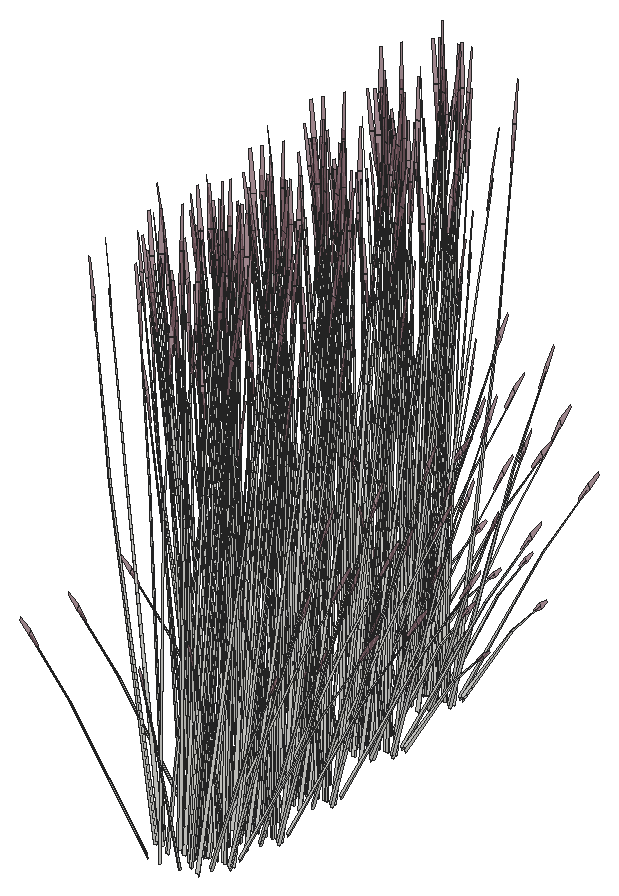
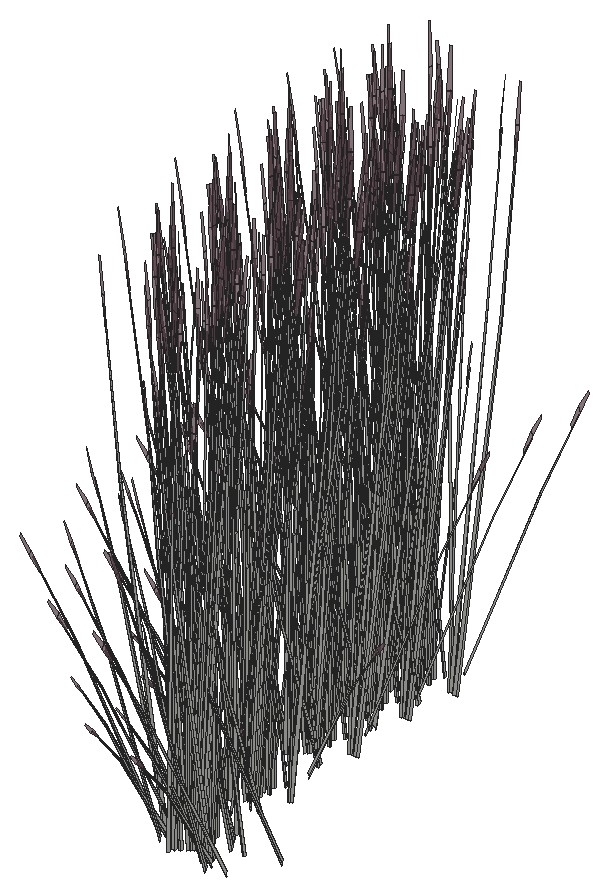
# SketchUp Ruby script. Lengths in inches.
U = 1.inch
M = Sketchup.active_model
def pt(a) = Geom::Point3d.new(a.map { |v| v * U })
def face(e, loops, mat)
  f = e.add_face(loops[0].map { |a| pt(a) })
  loops[1..].each { |l| e.add_face(l.map { |a| pt(a) }).erase! }
  f.material = f.back_material = mat if mat
  f
end
# faces: each face lists its corners as indices into pts; further lists are holes
def faces(e, pts, list, mat = nil) = list.each { |f| face(e, (f[0].is_a?(Array) ? f : [f]).map { |l| l.map { |i| pts[i] } }, mat) }
# xy, xz, yz: faces in a plane at the given z, y or x. An outline is a flat list of corners, or four numbers for a rectangle; further outlines are holes
def ring(l) = l.size == 4 ? [[l[0], l[1]], [l[2], l[1]], [l[2], l[3]], [l[0], l[3]]] : l.each_slice(2).to_a
def flat(e, list, mat, &to3) = list.each { |f| face(e, (f[0].is_a?(Array) ? f : [f]).map { |l| ring(l).map { |u, v| to3.(u, v) } }, mat) }
def xy(e, z, list, mat = nil) = flat(e, list, mat) { |x, y| [x, y, z] }
def xz(e, y, list, mat = nil) = flat(e, list, mat) { |x, z| [x, y, z] }
def yz(e, x, list, mat = nil) = flat(e, list, mat) { |y, z| [x, y, z] }
def lines(e, pts, list) = list.each { |a, b| e.add_line(pt(pts[a]), pt(pts[b])) }
# prism: a flat outline (further loops are holes) pulled along v
def prism(e, loops, v, mat = nil)
  f = face(e, loops, mat); d = Geom::Vector3d.new(v.map { |x| x * U })
  f.pushpull(f.normal.samedirection?(d) ? d.length : -d.length)
end
def box(e, o, s, mat = nil) = prism(e, [[o, [o[0] + s[0], o[1], o[2]], [o[0] + s[0], o[1] + s[1], o[2]], [o[0], o[1] + s[1], o[2]]]], [0, 0, s[2]], mat)
def at(x, y, z, deg = 0) = Geom::Transformation.translation(pt([x, y, z])) * Geom::Transformation.rotation(ORIGIN, Z_AXIS, deg.degrees)
def axes(o, x, y, z) = Geom::Transformation.new([*x, 0, *y, 0, *z, 0, *pt(o).to_a, 1])
def part(name) = M.definitions.add(name)
# library, detail: a bought-in or finely detailed component or shape, given as its bounding box
def library(name, o, s) = part(name).tap { |d| box(d.entities, o, s) }
def detail(e, o, s) = box(e.add_group.entities, o, s)
def put(e, d, t, mat = nil) = e.add_instance(d, t).tap { |i| i.material = mat if mat }
def group(e, t, mat = nil) = e.add_group.tap { |g| g.transformation = t; g.material = mat if mat }.entities
root = M.entities
M.materials.add("LightPink_Translucent").color = [144, 107, 117]
M.materials["LightPink_Translucent"].alpha = 0.75
c1 = part("blade")
p = [[2.15,0.21,22],[0,0.17,0],[0.09,0.45,0],[2.18,0.31,22],[2.29,0.31,22],[0.38,0.45,0],
  [2.48,0.24,33],[2.49,0.24,33],[2.48,0.22,33]]
faces(c1.entities,p,[[0,1,2,3],[4,5,2,3],[6,3,4,7],[8,0,3,6]])
c2 = part("seeds")
p = [[0.3,-0.1,1.38],[-0.01,-0.03,1.59],[-0.01,-0.03,0.03],[0.14,-0.07,-0.07],[0.29,-0.03,3],[0.15,0.01,3.11]]
faces(c2.entities,p,[[0,1,2,3],[1,0,4,5]],"LightPink_Translucent")
c3 = part("blade with seeds")
put(c3.entities,c1,at(0,0,0))
put(c3.entities,c2,axes([2.4,0.25,30.99],[1.5799,-0.05474,1.17369],[-0.12525,1.92788,0.29478],[-0.07173,-0.02425,1.56792]))
put(root,c3,axes([684.41,330.09,265.93],[-0.60515,0.48003,0.25528],[-0.60552,-0.47498,-0.30288],[-0.02113,-0.13632,1.36855]))
put(root,c3,axes([686.64,317.69,265.97],[-0.40676,0.57214,0],[-0.68052,-0.31907,-0.42834],[-0.15499,-0.07267,1.3588]))
put(root,c3,axes([685.4375,325.0625,266.15],[0.2053,-0.09007,1.18691],[0.50689,0.27159,-0.25526],[-0.15087,0.235,0.50747]))
put(root,c3,axes([685.47,313.58,266.15],[0.2053,-0.09007,1.18691],[0.50689,0.27159,-0.25526],[-0.15087,0.235,0.50747]))
put(root,c3,axes([684.76,327.24,266.3],[0.33937,0.19872,0.95334],[-0.49424,0.11946,0.70045],[-0.10575,-0.15273,0.20998]))
put(root,c3,axes([683.1875,341.02,266.34],[0.59102,-0.10111,0.05401],[0.13587,0.40735,-0.71633],[-0.03747,0.2062,0.64209]))
put(root,c3,axes([686.01,319.34,266.15],[-0.0394,0.18678,1.18691],[-0.57594,0.15636,-0.25526],[-0.13463,-0.24142,0.50747]))
put(root,c3,axes([686.04,307.86,266.15],[-0.0394,0.18678,1.18691],[-0.57594,0.15636,-0.25526],[-0.13463,-0.24142,0.50747]))
put(root,c3,axes([684.875,333.56,266.3],[-0.01684,-0.3395,0.95334],[0.42072,0.24214,0.70045],[-0.08274,0.16182,0.20998]))
put(root,c3,axes([685.89,318.52,266.15],[0.2053,-0.09007,1.18691],[0.50689,0.27159,-0.25526],[-0.15087,0.235,0.50747]))
put(root,c3,axes([684.84,322.06,265.97],[-0.81352,0,0],[0,-0.63814,-0.42834],[0,-0.14534,1.3588]))
put(root,c3,axes([684.87,310.57,265.97],[-0.81352,0,0],[0,-0.63814,-0.42834],[0,-0.14534,1.3588]))
put(root,c3,axes([685.47,332.14,266.06],[0.60889,0.28548,0.4121],[-0.36394,0.51192,0],[-0.13868,-0.06502,1.30728]))
put(root,c3,axes([681.9,341.89,266.3],[-0.36631,-0.16417,0.95334],[0.47299,-0.16681,0.70045],[0.12758,0.1413,0.20998]))
put(root,c3,axes([684.8,338.95,265.96],[0.82229,0.1203,0.37976],[-0.16734,0.67942,0.14902],[-0.12017,-0.06561,1.31851]))
put(root,c3,axes([680.6,341.72,266.15],[0.01148,-0.18927,1.18691],[0.54864,-0.21141,-0.25526],[0.16937,0.22654,0.50747]))
put(root,c3,axes([686.46,312.8,266.15],[-0.0394,0.18678,1.18691],[-0.57594,0.15636,-0.25526],[-0.13463,-0.24142,0.50747]))
put(root,c3,axes([684.59,338.83,266.26],[-0.31565,0.51449,0.37133],[-0.65588,-0.24761,-0.17871],[0,-0.1186,1.19224]))
put(root,c3,axes([686.35,331.25,266.17],[-0.12551,0.50956,0.12018],[-0.6132,-0.08845,-0.34318],[-0.1116,-0.05232,1.05198]))
put(root,c3,axes([685.47,321.89,265.93],[-0.60515,0.48003,0.25528],[-0.60552,-0.47498,-0.30288],[-0.02113,-0.13632,1.36855]))
put(root,c3,axes([685.29,315.51,265.97],[-0.81352,0,0],[0,-0.63814,-0.42834],[0,-0.14534,1.3588]))
put(root,c3,axes([685.5,310.4,265.93],[-0.60515,0.48003,0.25528],[-0.60552,-0.47498,-0.30288],[-0.02113,-0.13632,1.36855]))
put(root,c3,axes([684.27,330.35,266.06],[0,0.57097,0.4121],[-0.72788,0,0],[0,-0.13004,1.30728]))
put(root,c3,axes([687.61,332.51,265.82],[-0.40169,-0.57414,-0.04268],[0.68052,-0.31907,0.42834],[-0.16769,0.05466,1.35813]))
put(root,c3,axes([678.58,338.1,266.15],[-0.15668,-0.14043,1.18691],[0.20386,-0.46454,-0.25526],[0.31701,0.06293,0.50747]))
put(root,c3,axes([683.01,340.28,265.97],[0.81352,0,0],[0,0.63814,-0.42834],[0,0.14534,1.3588]))
put(root,c3,axes([684.36,340.04,266.05],[0.6991,-0.15154,0.14643],[0.17263,0.56398,0.29122],[-0.06235,-0.08217,1.33138]))
put(root,c3,axes([685.26,340.125,265.82],[-0.65588,-0.25634,0],[0.31565,-0.53263,0],[0,0,1.35047]))
put(root,c3,axes([681.96,342.64,266.21],[-0.4172,-0.01791,0.872],[0.27552,-0.38032,0.48145],[0.16481,0.13512,0.68401]))
put(root,c3,axes([686.78,340.77,265.97],[0.40676,0.57214,0],[-0.68052,0.31907,-0.42834],[-0.15499,0.07267,1.3588]))
put(root,c3,axes([685.92,315.35,265.93],[-0.60515,0.48003,0.25528],[-0.60552,-0.47498,-0.30288],[-0.02113,-0.13632,1.36855]))
put(root,c3,axes([686.44,340.07,266.05],[0.18794,-0.56744,0.14643],[0.68774,0.16058,0.29122],[-0.1188,0.00276,1.33138]))
put(root,c3,axes([686.125,339.3125,266.17],[0.48065,0.34305,0.12018],[-0.40092,0.38703,-0.34318],[-0.1116,0.05232,1.05198]))
put(root,c3,axes([684.52,332.83,266.34],[0.59102,-0.10111,0.05401],[0.13587,0.40735,-0.71633],[-0.03747,0.2062,0.64209]))
put(root,c3,axes([686.53,323.9375,266.06],[0.60889,0.28548,0.4121],[-0.36394,0.51192,0],[-0.13868,-0.06502,1.30728]))
put(root,c3,axes([685.95,338.89,265.91],[-0.60515,-0.49144,-0.05089],[0.60552,-0.49174,0],[-0.02113,-0.01716,1.45724]))
put(root,c3,axes([686.5625,312.45,266.06],[0.60889,0.28548,0.4121],[-0.36394,0.51192,0],[-0.13868,-0.06502,1.30728]))
put(root,c3,axes([686.11,339.0625,266.26],[0.70648,-0.03525,0.37133],[0.06389,0.58508,-0.17871],[-0.12647,0.0593,1.19224]))
put(root,c3,axes([686.29,340.41,265.93],[0.81449,0.18558,0.25528],[-0.20377,0.66335,-0.30288],[-0.13481,0.08302,1.36855]))
put(root,c3,axes([687.4,323.05,266.17],[-0.12551,0.50956,0.12018],[-0.6132,-0.08845,-0.34318],[-0.1116,-0.05232,1.05198]))
put(root,c3,axes([686.64,340.37,266.06],[0.60889,-0.28548,0.4121],[0.36394,0.51192,0],[-0.13868,0.06502,1.30728]))
put(root,c3,axes([687.4375,311.5625,266.17],[-0.12551,0.50956,0.12018],[-0.6132,-0.08845,-0.34318],[-0.1116,-0.05232,1.05198]))
put(root,c3,axes([686.14,330.76,265.96],[0.82229,0.1203,0.37976],[-0.16734,0.67942,0.14902],[-0.12017,-0.06561,1.31851]))
put(root,c3,axes([684.73,338.33,265.96],[0.28286,0.63846,0.37976],[-0.80821,0.22202,0.14902],[0.00988,-0.11732,1.31851]))
put(root,c3,axes([685.33,322.15,266.06],[0,0.57097,0.4121],[-0.72788,0,0],[0,-0.13004,1.30728]))
put(root,c3,axes([688.66,324.3125,265.82],[-0.40169,-0.57414,-0.04268],[0.68052,-0.31907,0.42834],[-0.16769,0.05466,1.35813]))
put(root,c3,axes([681.66,338.1,265.97],[0.40676,-0.57214,0],[0.68052,0.31907,-0.42834],[0.15499,0.07267,1.3588]))
put(root,c3,axes([685.36,310.67,266.06],[0,0.57097,0.4121],[-0.72788,0,0],[0,-0.13004,1.30728]))
put(root,c3,axes([688.7,312.83,265.82],[-0.40169,-0.57414,-0.04268],[0.68052,-0.31907,0.42834],[-0.16769,0.05466,1.35813]))
put(root,c3,axes([685.41,339.9,265.83],[-0.21227,-0.49226,0],[0.60616,-0.17239,0],[0,0,1.28128]))
put(root,c3,axes([686.99,317.39,266.06],[0.60889,0.28548,0.4121],[-0.36394,0.51192,0],[-0.13868,-0.06502,1.30728]))
put(root,c3,axes([685.93,330.64,266.26],[-0.31565,0.51449,0.37133],[-0.65588,-0.24761,-0.17871],[0,-0.1186,1.19224]))
put(root,c3,axes([687.86,316.51,266.17],[-0.12551,0.50956,0.12018],[-0.6132,-0.08845,-0.34318],[-0.1116,-0.05232,1.05198]))
put(root,c3,axes([685.7,331.85,266.05],[0.6991,-0.15154,0.14643],[0.17263,0.56398,0.29122],[-0.06235,-0.08217,1.33138]))
put(root,c3,axes([685.79,315.61,266.06],[0,0.57097,0.4121],[-0.72788,0,0],[0,-0.13004,1.30728]))
put(root,c3,axes([689.12,317.77,265.82],[-0.40169,-0.57414,-0.04268],[0.68052,-0.31907,0.42834],[-0.16769,0.05466,1.35813]))
put(root,c3,axes([686.6,331.9375,265.82],[-0.65588,-0.25634,0],[0.31565,-0.53263,0],[0,0,1.35047]))
put(root,c3,axes([688.12,332.58,265.97],[0.40676,0.57214,0],[-0.68052,0.31907,-0.42834],[-0.15499,0.07267,1.3588]))
put(root,c3,axes([685.58,324.63,266.34],[0.59102,-0.10111,0.05401],[0.13587,0.40735,-0.71633],[-0.03747,0.2062,0.64209]))
put(root,c3,axes([685.61,313.15,266.34],[0.59102,-0.10111,0.05401],[0.13587,0.40735,-0.71633],[-0.03747,0.2062,0.64209]))
put(root,c3,axes([687.52,338.62,266.05],[-0.51116,-0.4159,0.14643],[0.51512,-0.4034,0.29122],[-0.05645,0.08494,1.33138]))
put(root,c3,axes([685.75,338.38,265.83],[0,-0.66065,0],[0.81352,0,0],[0,0,1.48949]))
put(root,c3,axes([685,338.5,266.02],[0.73304,0.27674,0.19974],[-0.35279,0.57501,0.41502],[0,-0.13255,1.3325]))
put(root,c3,axes([683.1,338.02,266.3],[-0.2167,0.29065,0.95334],[-0.18626,-0.3905,0.70045],[0.17898,-0.09785,0.20998]))
put(root,c3,axes([686.16,338.64,265.9],[0,0.66033,-0.04679],[-0.81352,0,0],[0,0.02075,1.48875]))
put(root,c3,axes([684.76,338.11,266.26],[-0.70648,0.03525,0.37133],[-0.06389,-0.58508,-0.17871],[0.12647,-0.0593,1.19224]))
put(root,c3,axes([687.78,331.88,266.05],[0.18794,-0.56744,0.14643],[0.68774,0.16058,0.29122],[-0.1188,0.00276,1.33138]))
put(root,c3,axes([687.47,331.125,266.17],[0.48065,0.34305,0.12018],[-0.40092,0.38703,-0.34318],[-0.1116,0.05232,1.05198]))
put(root,c3,axes([687.29,330.7,265.91],[-0.60515,-0.49144,-0.05089],[0.60552,-0.49174,0],[-0.02113,-0.01716,1.45724]))
put(root,c3,axes([684.43,337.11,266.05],[-0.18794,0.56744,0.14643],[-0.68774,-0.16058,0.29122],[0.1188,-0.00276,1.33138]))
put(root,c3,axes([687.2,322.5625,265.96],[0.82229,0.1203,0.37976],[-0.16734,0.67942,0.14902],[-0.12017,-0.06561,1.31851]))
put(root,c3,axes([685.77,339.92,265.9],[0.28286,0.65594,-0.0499],[-0.80821,0.22985,0],[0.00988,0.02291,1.42904]))
put(root,c3,axes([687.45,330.875,266.26],[0.70648,-0.03525,0.37133],[0.06389,0.58508,-0.17871],[-0.12647,0.0593,1.19224]))
put(root,c3,axes([687.23,311.08,265.96],[0.82229,0.1203,0.37976],[-0.16734,0.67942,0.14902],[-0.12017,-0.06561,1.31851]))
put(root,c3,axes([686.04,318.09,266.34],[0.59102,-0.10111,0.05401],[0.13587,0.40735,-0.71633],[-0.03747,0.2062,0.64209]))
put(root,c3,axes([687.625,332.22,265.93],[0.81449,0.18558,0.25528],[-0.20377,0.66335,-0.30288],[-0.13481,0.08302,1.36855]))
put(root,c3,axes([686.99,322.44,266.26],[-0.31565,0.51449,0.37133],[-0.65588,-0.24761,-0.17871],[0,-0.1186,1.19224]))
put(root,c3,axes([687.98,332.18,266.06],[0.60889,-0.28548,0.4121],[0.36394,0.51192,0],[-0.13868,0.06502,1.30728]))
put(root,c3,axes([687.02,310.96,266.26],[-0.31565,0.51449,0.37133],[-0.65588,-0.24761,-0.17871],[0,-0.1186,1.19224]))
put(root,c3,axes([684.09,336.41,265.97],[-0.40676,-0.57214,0],[0.68052,-0.31907,-0.42834],[0.15499,-0.07267,1.3588]))
put(root,c3,axes([688.11,339.06,265.83],[-0.81312,-0.00457,-0.0413],[0,-0.63814,0.41452],[-0.02555,0.14527,1.31432]))
put(root,c3,axes([686.07,330.14,265.96],[0.28286,0.63846,0.37976],[-0.80821,0.22202,0.14902],[0.00988,-0.11732,1.31851]))
put(root,c3,axes([686.75,331.72,265.83],[-0.21227,-0.49226,0],[0.60616,-0.17239,0],[0,0,1.28128]))
put(root,c3,axes([686.51,337.14,266.05],[-0.6991,0.15154,0.14643],[-0.17263,-0.56398,0.29122],[0.06235,0.08217,1.33138]))
put(root,c3,axes([687.66,316.02,265.96],[0.82229,0.1203,0.37976],[-0.16734,0.67942,0.14902],[-0.12017,-0.06561,1.31851]))
put(root,c3,axes([686.76,323.65,266.05],[0.6991,-0.15154,0.14643],[0.17263,0.56398,0.29122],[-0.06235,-0.08217,1.33138]))
put(root,c3,axes([686.79,312.16,266.05],[0.6991,-0.15154,0.14643],[0.17263,0.56398,0.29122],[-0.06235,-0.08217,1.33138]))
put(root,c3,axes([685.8,335.03,266.3],[0.08346,0.33295,0.95334],[-0.46298,-0.1844,0.70045],[0.04982,-0.17048,0.20998]))
put(root,c3,axes([687.66,323.74,265.82],[-0.65588,-0.25634,0],[0.31565,-0.53263,0],[0,0,1.35047]))
put(root,c3,axes([685.37,337.96,265.96],[-0.53943,0.51816,0.37976],[-0.64086,-0.4574,0.14902],[0.13005,-0.05171,1.31851]))
put(root,c3,axes([687.69,312.25,265.82],[-0.65588,-0.25634,0],[0.31565,-0.53263,0],[0,0,1.35047]))
put(root,c3,axes([689.17,324.38,265.97],[0.40676,0.57214,0],[-0.68052,0.31907,-0.42834],[-0.15499,0.07267,1.3588]))
put(root,c3,axes([689.21,312.9,265.97],[0.40676,0.57214,0],[-0.68052,0.31907,-0.42834],[-0.15499,0.07267,1.3588]))
put(root,c3,axes([686.29,338.78,265.84],[0.45414,0.3688,0],[-0.45414,0.3688,0],[0,0,1.40491]))
put(root,c3,axes([687.44,315.9,266.26],[-0.31565,0.51449,0.37133],[-0.65588,-0.24761,-0.17871],[0,-0.1186,1.19224]))
put(root,c3,axes([686.28,338.35,266.26],[0.31565,-0.51449,0.37133],[0.65588,0.24761,-0.17871],[0,0.1186,1.19224]))
put(root,c3,axes([686.01,340.14,265.83],[0.65588,0.25634,0],[-0.31565,0.53263,0],[0,0,1.45212]))
put(root,c3,axes([686.07,338.23,265.98],[-0.82229,-0.1203,0.40835],[0.16734,-0.67942,0.16024],[0.12017,0.06561,1.41775]))
put(root,c3,axes([688.84,323.68,266.05],[0.18794,-0.56744,0.14643],[0.68774,0.16058,0.29122],[-0.1188,0.00276,1.33138]))
put(root,c3,axes([688.52,322.93,266.17],[0.48065,0.34305,0.12018],[-0.40092,0.38703,-0.34318],[-0.1116,0.05232,1.05198]))
put(root,c3,axes([687.21,317.11,266.05],[0.6991,-0.15154,0.14643],[0.17263,0.56398,0.29122],[-0.06235,-0.08217,1.33138]))
put(root,c3,axes([688.87,312.2,266.05],[0.18794,-0.56744,0.14643],[0.68774,0.16058,0.29122],[-0.1188,0.00276,1.33138]))
put(root,c3,axes([688.55,311.44,266.17],[0.48065,0.34305,0.12018],[-0.40092,0.38703,-0.34318],[-0.1116,0.05232,1.05198]))
put(root,c3,axes([688.86,330.43,266.05],[-0.51116,-0.4159,0.14643],[0.51512,-0.4034,0.29122],[-0.05645,0.08494,1.33138]))
put(root,c3,axes([688.35,322.5,265.91],[-0.60515,-0.49144,-0.05089],[0.60552,-0.49174,0],[-0.02113,-0.01716,1.45724]))
put(root,c3,axes([688.11,317.2,265.82],[-0.65588,-0.25634,0],[0.31565,-0.53263,0],[0,0,1.35047]))
put(root,c3,axes([688.51,322.67,266.26],[0.70648,-0.03525,0.37133],[0.06389,0.58508,-0.17871],[-0.12647,0.0593,1.19224]))
put(root,c3,axes([688.38,311.02,265.91],[-0.60515,-0.49144,-0.05089],[0.60552,-0.49174,0],[-0.02113,-0.01716,1.45724]))
put(root,c3,axes([687.09,330.19,265.83],[0,-0.66065,0],[0.81352,0,0],[0,0,1.48949]))
put(root,c3,axes([689.63,317.84,265.97],[0.40676,0.57214,0],[-0.68052,0.31907,-0.42834],[-0.15499,0.07267,1.3588]))
put(root,c3,axes([688.54,311.19,266.26],[0.70648,-0.03525,0.37133],[0.06389,0.58508,-0.17871],[-0.12647,0.0593,1.19224]))
put(root,c3,axes([686.33,330.3125,266.02],[0.73304,0.27674,0.19974],[-0.35279,0.57501,0.41502],[0,-0.13255,1.3325]))
put(root,c3,axes([687.5,330.45,265.9],[0,0.66033,-0.04679],[-0.81352,0,0],[0,0.02075,1.48875]))
put(root,c3,axes([686.3,338.53,265.83],[0.72788,0,0],[0,0.59111,0],[0,0,1.48078]))
put(root,c3,axes([686.1,329.93,266.26],[-0.70648,0.03525,0.37133],[-0.06389,-0.58508,-0.17871],[0.12647,-0.0593,1.19224]))
put(root,c3,axes([688.68,324.02,265.93],[0.81449,0.18558,0.25528],[-0.20377,0.66335,-0.30288],[-0.13481,0.08302,1.36855]))
put(root,c3,axes([688.71,312.54,265.93],[0.81449,0.18558,0.25528],[-0.20377,0.66335,-0.30288],[-0.13481,0.08302,1.36855]))
put(root,c3,axes([685.6,337.875,266.26],[-0.39083,-0.47924,0.37133],[0.59199,-0.33747,-0.17871],[0.12647,0.0593,1.19224]))
put(root,c3,axes([684.14,340.54,266.3],[-0.40197,0.09426,0.95334],[0.18921,-0.38956,0.70045],[0.21325,0.02666,0.20998]))
put(root,c3,axes([686.56,338.47,266.17],[0.60616,-0.16651,0.12018],[0.21227,0.47548,-0.34318],[0,0.10465,1.05198]))
put(root,c3,axes([689.03,323.98,266.06],[0.60889,-0.28548,0.4121],[0.36394,0.51192,0],[-0.13868,0.06502,1.30728]))
put(root,c3,axes([685.77,328.92,266.05],[-0.18794,0.56744,0.14643],[-0.68774,-0.16058,0.29122],[0.1188,-0.00276,1.33138]))
put(root,c3,axes([689.07,312.5,266.06],[0.60889,-0.28548,0.4121],[0.36394,0.51192,0],[-0.13868,0.06502,1.30728]))
put(root,c3,axes([687.11,331.73,265.9],[0.28286,0.65594,-0.0499],[-0.80821,0.22985,0],[0.00988,0.02291,1.42904]))
put(root,c3,axes([687.13,321.9375,265.96],[0.28286,0.63846,0.37976],[-0.80821,0.22202,0.14902],[0.00988,-0.11732,1.31851]))
put(root,c3,axes([689.29,317.14,266.05],[0.18794,-0.56744,0.14643],[0.68774,0.16058,0.29122],[-0.1188,0.00276,1.33138]))
put(root,c3,axes([688.98,316.38,266.17],[0.48065,0.34305,0.12018],[-0.40092,0.38703,-0.34318],[-0.1116,0.05232,1.05198]))
put(root,c3,axes([687.16,310.45,265.96],[0.28286,0.63846,0.37976],[-0.80821,0.22202,0.14902],[0.00988,-0.11732,1.31851]))
put(root,c3,axes([682.83,338.85,266.15],[-0.23242,-0.01691,1.18691],[-0.23811,-0.45367,-0.25526],[0.28553,-0.12834,0.50747]))
put(root,c3,axes([687.81,323.51,265.83],[-0.21227,-0.49226,0],[0.60616,-0.17239,0],[0,0,1.28128]))
put(root,c3,axes([687.84,312.03,265.83],[-0.21227,-0.49226,0],[0.60616,-0.17239,0],[0,0,1.28128]))
put(root,c3,axes([688.81,315.96,265.91],[-0.60515,-0.49144,-0.05089],[0.60552,-0.49174,0],[-0.02113,-0.01716,1.45724]))
put(root,c3,axes([688.97,316.13,266.26],[0.70648,-0.03525,0.37133],[0.06389,0.58508,-0.17871],[-0.12647,0.0593,1.19224]))
put(root,c3,axes([685.43,328.22,265.97],[-0.40676,-0.57214,0],[0.68052,-0.31907,-0.42834],[0.15499,-0.07267,1.3588]))
put(root,c3,axes([689.45,330.87,265.83],[-0.81312,-0.00457,-0.0413],[0,-0.63814,0.41452],[-0.02555,0.14527,1.31432]))
put(root,c3,axes([689.14,317.48,265.93],[0.81449,0.18558,0.25528],[-0.20377,0.66335,-0.30288],[-0.13481,0.08302,1.36855]))
put(root,c3,axes([689.49,317.44,266.06],[0.60889,-0.28548,0.4121],[0.36394,0.51192,0],[-0.13868,0.06502,1.30728]))
put(root,c3,axes([687.85,328.95,266.05],[-0.6991,0.15154,0.14643],[-0.17263,-0.56398,0.29122],[0.06235,0.08217,1.33138]))
put(root,c3,axes([686.48,335.95,266.15],[-0.18493,0.11557,1.18691],[-0.55384,-0.20228,-0.25526],[0.10266,-0.25157,0.50747]))
put(root,c3,axes([683.26,340.36,265.65],[-0.41902,0.06852,1.17514],[-0.0667,-0.54541,0.06726],[0.29348,-0.08255,0.6687]))
put(root,c3,axes([687.58,315.4,265.96],[0.28286,0.63846,0.37976],[-0.80821,0.22202,0.14902],[0.00988,-0.11732,1.31851]))
put(root,c3,axes([687.14,326.84,266.3],[0.08346,0.33295,0.95334],[-0.46298,-0.1844,0.70045],[0.04982,-0.17048,0.20998]))
put(root,c3,axes([688.26,316.97,265.83],[-0.21227,-0.49226,0],[0.60616,-0.17239,0],[0,0,1.28128]))
put(root,c3,axes([687.9375,338.64,266.06],[0,-0.57097,0.4121],[0.72788,0,0],[0,0.13004,1.30728]))
put(root,c3,axes([686.71,329.77,265.96],[-0.53943,0.51816,0.37976],[-0.64086,-0.4574,0.14902],[0.13005,-0.05171,1.31851]))
put(root,c3,axes([687.625,330.59,265.84],[0.45414,0.3688,0],[-0.45414,0.3688,0],[0,0,1.40491]))
put(root,c3,axes([685.87,337.74,266.17],[0.12551,-0.50956,0.12018],[0.6132,0.08845,-0.34318],[0.1116,0.05232,1.05198]))
put(root,c3,axes([687.62,330.16,266.26],[0.31565,-0.51449,0.37133],[0.65588,0.24761,-0.17871],[0,0.1186,1.19224]))
put(root,c3,axes([687.35,331.95,265.83],[0.65588,0.25634,0],[-0.31565,0.53263,0],[0,0,1.45212]))
put(root,c3,axes([689.91,322.23,266.05],[-0.51116,-0.4159,0.14643],[0.51512,-0.4034,0.29122],[-0.05645,0.08494,1.33138]))
put(root,c3,axes([689.95,310.75,266.05],[-0.51116,-0.4159,0.14643],[0.51512,-0.4034,0.29122],[-0.05645,0.08494,1.33138]))
put(root,c3,axes([688.15,321.99,265.83],[0,-0.66065,0],[0.81352,0,0],[0,0,1.48949]))
put(root,c3,axes([688.18,310.51,265.83],[0,-0.66065,0],[0.81352,0,0],[0,0,1.48949]))
put(root,c3,axes([687.39,322.11,266.02],[0.73304,0.27674,0.19974],[-0.35279,0.57501,0.41502],[0,-0.13255,1.3325]))
put(root,c3,axes([688.55,322.25,265.9],[0,0.66033,-0.04679],[-0.81352,0,0],[0,0.02075,1.48875]))
put(root,c3,axes([687.42,310.63,266.02],[0.73304,0.27674,0.19974],[-0.35279,0.57501,0.41502],[0,-0.13255,1.3325]))
put(root,c3,axes([687.15,321.73,266.26],[-0.70648,0.03525,0.37133],[-0.06389,-0.58508,-0.17871],[0.12647,-0.0593,1.19224]))
put(root,c3,axes([688.59,310.77,265.9],[0,0.66033,-0.04679],[-0.81352,0,0],[0,0.02075,1.48875]))
put(root,c3,axes([687.41,330.04,265.98],[-0.82229,-0.1203,0.40835],[0.16734,-0.67942,0.16024],[0.12017,0.06561,1.41775]))
put(root,c3,axes([687.1875,310.24,266.26],[-0.70648,0.03525,0.37133],[-0.06389,-0.58508,-0.17871],[0.12647,-0.0593,1.19224]))
put(root,c3,axes([686.74,336.85,266.06],[-0.60889,-0.28548,0.4121],[0.36394,-0.51192,0],[0.13868,0.06502,1.30728]))
put(root,c3,axes([686.82,320.72,266.05],[-0.18794,0.56744,0.14643],[-0.68774,-0.16058,0.29122],[0.1188,-0.00276,1.33138]))
put(root,c3,axes([688.17,323.53,265.9],[0.28286,0.65594,-0.0499],[-0.80821,0.22985,0],[0.00988,0.02291,1.42904]))
put(root,c3,axes([686.86,309.24,266.05],[-0.18794,0.56744,0.14643],[-0.68774,-0.16058,0.29122],[0.1188,-0.00276,1.33138]))
put(root,c3,axes([688.2,312.05,265.9],[0.28286,0.65594,-0.0499],[-0.80821,0.22985,0],[0.00988,0.02291,1.42904]))
put(root,c3,axes([687.64,330.34,265.83],[0.72788,0,0],[0,0.59111,0],[0,0,1.48078]))
put(root,c3,axes([690.37,315.69,266.05],[-0.51116,-0.4159,0.14643],[0.51512,-0.4034,0.29122],[-0.05645,0.08494,1.33138]))
put(root,c3,axes([688.6,315.45,265.83],[0,-0.66065,0],[0.81352,0,0],[0,0,1.48949]))
put(root,c3,axes([686.94,329.6875,266.26],[-0.39083,-0.47924,0.37133],[0.59199,-0.33747,-0.17871],[0.12647,0.0593,1.19224]))
put(root,c3,axes([687.89,330.28,266.17],[0.60616,-0.16651,0.12018],[0.21227,0.47548,-0.34318],[0,0.10465,1.05198]))
put(root,c3,axes([687.85,315.57,266.02],[0.73304,0.27674,0.19974],[-0.35279,0.57501,0.41502],[0,-0.13255,1.3325]))
put(root,c3,axes([689.01,315.71,265.9],[0,0.66033,-0.04679],[-0.81352,0,0],[0,0.02075,1.48875]))
put(root,c3,axes([686.49,320.02,265.97],[-0.40676,-0.57214,0],[0.68052,-0.31907,-0.42834],[0.15499,-0.07267,1.3588]))
put(root,c3,axes([690.5,322.67,265.83],[-0.81312,-0.00457,-0.0413],[0,-0.63814,0.41452],[-0.02555,0.14527,1.31432]))
put(root,c3,axes([687.61,315.18,266.26],[-0.70648,0.03525,0.37133],[-0.06389,-0.58508,-0.17871],[0.12647,-0.0593,1.19224]))
put(root,c3,axes([686.52,308.54,265.97],[-0.40676,-0.57214,0],[0.68052,-0.31907,-0.42834],[0.15499,-0.07267,1.3588]))
put(root,c3,axes([690.54,311.1875,265.83],[-0.81312,-0.00457,-0.0413],[0,-0.63814,0.41452],[-0.02555,0.14527,1.31432]))
put(root,c3,axes([683.38,341.17,266.15],[-0.15668,-0.14043,1.18691],[0.20386,-0.46454,-0.25526],[0.31701,0.06293,0.50747]))
put(root,c3,axes([688.9,320.75,266.05],[-0.6991,0.15154,0.14643],[-0.17263,-0.56398,0.29122],[0.06235,0.08217,1.33138]))
put(root,c3,axes([687.28,314.18,266.05],[-0.18794,0.56744,0.14643],[-0.68774,-0.16058,0.29122],[0.1188,-0.00276,1.33138]))
put(root,c3,axes([688.9375,309.27,266.05],[-0.6991,0.15154,0.14643],[-0.17263,-0.56398,0.29122],[0.06235,0.08217,1.33138]))
put(root,c3,axes([688.62,316.99,265.9],[0.28286,0.65594,-0.0499],[-0.80821,0.22985,0],[0.00988,0.02291,1.42904]))
put(root,c3,axes([687.76,321.57,265.96],[-0.53943,0.51816,0.37976],[-0.64086,-0.4574,0.14902],[0.13005,-0.05171,1.31851]))
put(root,c3,axes([687.33,340.35,266.3],[-0.36631,-0.16417,0.95334],[0.47299,-0.16681,0.70045],[0.12758,0.1413,0.20998]))
put(root,c3,axes([686.02,340.17,266.15],[0.01148,-0.18927,1.18691],[0.54864,-0.21141,-0.25526],[0.16937,0.22654,0.50747]))
put(root,c3,axes([687.79,310.09,265.96],[-0.53943,0.51816,0.37976],[-0.64086,-0.4574,0.14902],[0.13005,-0.05171,1.31851]))
put(root,c3,axes([688.68,322.39,265.84],[0.45414,0.3688,0],[-0.45414,0.3688,0],[0,0,1.40491]))
put(root,c3,axes([688.68,321.96,266.26],[0.31565,-0.51449,0.37133],[0.65588,0.24761,-0.17871],[0,0.1186,1.19224]))
put(root,c3,axes([688.72,310.91,265.84],[0.45414,0.3688,0],[-0.45414,0.3688,0],[0,0,1.40491]))
put(root,c3,axes([688.4,323.75,265.83],[0.65588,0.25634,0],[-0.31565,0.53263,0],[0,0,1.45212]))
put(root,c3,axes([687.82,327.76,266.15],[-0.18493,0.11557,1.18691],[-0.55384,-0.20228,-0.25526],[0.10266,-0.25157,0.50747]))
put(root,c3,axes([688.71,310.48,266.26],[0.31565,-0.51449,0.37133],[0.65588,0.24761,-0.17871],[0,0.1186,1.19224]))
put(root,c3,axes([686.94,313.48,265.97],[-0.40676,-0.57214,0],[0.68052,-0.31907,-0.42834],[0.15499,-0.07267,1.3588]))
put(root,c3,axes([688.44,312.26,265.83],[0.65588,0.25634,0],[-0.31565,0.53263,0],[0,0,1.45212]))
put(root,c3,axes([690.96,316.13,265.83],[-0.81312,-0.00457,-0.0413],[0,-0.63814,0.41452],[-0.02555,0.14527,1.31432]))
put(root,c3,axes([689.28,330.45,266.06],[0,-0.57097,0.4121],[0.72788,0,0],[0,0.13004,1.30728]))
put(root,c3,axes([689.36,314.21,266.05],[-0.6991,0.15154,0.14643],[-0.17263,-0.56398,0.29122],[0.06235,0.08217,1.33138]))
put(root,c3,axes([688.46,321.84,265.98],[-0.82229,-0.1203,0.40835],[0.16734,-0.67942,0.16024],[0.12017,0.06561,1.41775]))
put(root,c3,axes([688.5,310.35,265.98],[-0.82229,-0.1203,0.40835],[0.16734,-0.67942,0.16024],[0.12017,0.06561,1.41775]))
put(root,c3,axes([687.2,329.55,266.17],[0.12551,-0.50956,0.12018],[0.6132,0.08845,-0.34318],[0.1116,0.05232,1.05198]))
put(root,c3,axes([688.43,338.73,265.97],[0.81352,0,0],[0,0.63814,-0.42834],[0,0.14534,1.3588]))
put(root,c3,axes([688.22,315.03,265.96],[-0.53943,0.51816,0.37976],[-0.64086,-0.4574,0.14902],[0.13005,-0.05171,1.31851]))
put(root,c3,axes([689.14,315.85,265.84],[0.45414,0.3688,0],[-0.45414,0.3688,0],[0,0,1.40491]))
put(root,c3,axes([689.13,315.42,266.26],[0.31565,-0.51449,0.37133],[0.65588,0.24761,-0.17871],[0,0.1186,1.19224]))
put(root,c3,axes([688.86,317.21,265.83],[0.65588,0.25634,0],[-0.31565,0.53263,0],[0,0,1.45212]))
put(root,c3,axes([688.7,322.14,265.83],[0.72788,0,0],[0,0.59111,0],[0,0,1.48078]))
put(root,c3,axes([688.73,310.65,265.83],[0.72788,0,0],[0,0.59111,0],[0,0,1.48078]))
put(root,c3,axes([688.08,328.66,266.06],[-0.60889,-0.28548,0.4121],[0.36394,-0.51192,0],[0.13868,0.06502,1.30728]))
put(root,c3,axes([687.38,341.1,266.21],[-0.4172,-0.01791,0.872],[0.27552,-0.38032,0.48145],[0.16481,0.13512,0.68401]))
put(root,c3,axes([688,321.49,266.26],[-0.39083,-0.47924,0.37133],[0.59199,-0.33747,-0.17871],[0.12647,0.0593,1.19224]))
put(root,c3,axes([688.95,322.08,266.17],[0.60616,-0.16651,0.12018],[0.21227,0.47548,-0.34318],[0,0.10465,1.05198]))
put(root,c3,axes([688.03,310,266.26],[-0.39083,-0.47924,0.37133],[0.59199,-0.33747,-0.17871],[0.12647,0.0593,1.19224]))
put(root,c3,axes([688.98,310.59,266.17],[0.60616,-0.16651,0.12018],[0.21227,0.47548,-0.34318],[0,0.10465,1.05198]))
put(root,c3,axes([688.92,315.3,265.98],[-0.82229,-0.1203,0.40835],[0.16734,-0.67942,0.16024],[0.12017,0.06561,1.41775]))
put(root,c3,axes([689.15,315.6,265.83],[0.72788,0,0],[0,0.59111,0],[0,0,1.48078]))
put(root,c3,axes([688.45,314.95,266.26],[-0.39083,-0.47924,0.37133],[0.59199,-0.33747,-0.17871],[0.12647,0.0593,1.19224]))
put(root,c3,axes([689.41,315.54,266.17],[0.60616,-0.16651,0.12018],[0.21227,0.47548,-0.34318],[0,0.10465,1.05198]))
put(root,c3,axes([688.87,319.56,266.15],[-0.18493,0.11557,1.18691],[-0.55384,-0.20228,-0.25526],[0.10266,-0.25157,0.50747]))
put(root,c3,axes([688.91,308.07,266.15],[-0.18493,0.11557,1.18691],[-0.55384,-0.20228,-0.25526],[0.10266,-0.25157,0.50747]))
put(root,c3,axes([690.33,322.25,266.06],[0,-0.57097,0.4121],[0.72788,0,0],[0,0.13004,1.30728]))
put(root,c3,axes([690.37,310.76,266.06],[0,-0.57097,0.4121],[0.72788,0,0],[0,0.13004,1.30728]))
put(root,c3,axes([688.67,332.16,266.3],[-0.36631,-0.16417,0.95334],[0.47299,-0.16681,0.70045],[0.12758,0.1413,0.20998]))
put(root,c3,axes([687.36,331.99,266.15],[0.01148,-0.18927,1.18691],[0.54864,-0.21141,-0.25526],[0.16937,0.22654,0.50747]))
put(root,c3,axes([688.26,321.35,266.17],[0.12551,-0.50956,0.12018],[0.6132,0.08845,-0.34318],[0.1116,0.05232,1.05198]))
put(root,c3,axes([687.09,336.55,265.97],[0.40676,-0.57214,0],[0.68052,0.31907,-0.42834],[0.15499,0.07267,1.3588]))
put(root,c3,axes([688.29,309.87,266.17],[0.12551,-0.50956,0.12018],[0.6132,0.08845,-0.34318],[0.1116,0.05232,1.05198]))
put(root,c3,axes([689.33,313.02,266.15],[-0.18493,0.11557,1.18691],[-0.55384,-0.20228,-0.25526],[0.10266,-0.25157,0.50747]))
put(root,c3,axes([689.13,320.46,266.06],[-0.60889,-0.28548,0.4121],[0.36394,-0.51192,0],[0.13868,0.06502,1.30728]))
put(root,c3,axes([689.17,308.98,266.06],[-0.60889,-0.28548,0.4121],[0.36394,-0.51192,0],[0.13868,0.06502,1.30728]))
put(root,c3,axes([690.79,315.71,266.06],[0,-0.57097,0.4121],[0.72788,0,0],[0,0.13004,1.30728]))
put(root,c3,axes([689.77,330.54,265.97],[0.81352,0,0],[0,0.63814,-0.42834],[0,0.14534,1.3588]))
put(root,c3,axes([688.72,314.8125,266.17],[0.12551,-0.50956,0.12018],[0.6132,0.08845,-0.34318],[0.1116,0.05232,1.05198]))
put(root,c3,axes([688.72,332.91,266.21],[-0.4172,-0.01791,0.872],[0.27552,-0.38032,0.48145],[0.16481,0.13512,0.68401]))
put(root,c3,axes([689.59,313.92,266.06],[-0.60889,-0.28548,0.4121],[0.36394,-0.51192,0],[0.13868,0.06502,1.30728]))
put(root,c3,axes([688.53,336.47,266.3],[-0.2167,0.29065,0.95334],[-0.18626,-0.3905,0.70045],[0.17898,-0.09785,0.20998]))
put(root,c3,axes([688.42,323.79,266.15],[0.01148,-0.18927,1.18691],[0.54864,-0.21141,-0.25526],[0.16937,0.22654,0.50747]))
put(root,c3,axes([688.45,312.3,266.15],[0.01148,-0.18927,1.18691],[0.54864,-0.21141,-0.25526],[0.16937,0.22654,0.50747]))
put(root,c3,axes([688.43,328.37,265.97],[0.40676,-0.57214,0],[0.68052,0.31907,-0.42834],[0.15499,0.07267,1.3588]))
put(root,c3,axes([690.83,322.34,265.97],[0.81352,0,0],[0,0.63814,-0.42834],[0,0.14534,1.3588]))
put(root,c3,axes([690.86,310.86,265.97],[0.81352,0,0],[0,0.63814,-0.42834],[0,0.14534,1.3588]))
put(root,c3,axes([688.87,317.25,266.15],[0.01148,-0.18927,1.18691],[0.54864,-0.21141,-0.25526],[0.16937,0.22654,0.50747]))
put(root,c3,axes([689.78,324.71,266.21],[-0.4172,-0.01791,0.872],[0.27552,-0.38032,0.48145],[0.16481,0.13512,0.68401]))
put(root,c3,axes([689.8125,313.23,266.21],[-0.4172,-0.01791,0.872],[0.27552,-0.38032,0.48145],[0.16481,0.13512,0.68401]))
put(root,c3,axes([691.28,315.8,265.97],[0.81352,0,0],[0,0.63814,-0.42834],[0,0.14534,1.3588]))
put(root,c3,axes([690.23,318.17,266.21],[-0.4172,-0.01791,0.872],[0.27552,-0.38032,0.48145],[0.16481,0.13512,0.68401]))
put(root,c3,axes([689.87,328.29,266.3],[-0.2167,0.29065,0.95334],[-0.18626,-0.3905,0.70045],[0.17898,-0.09785,0.20998]))
put(root,c3,axes([689.5625,339,266.3],[-0.40197,0.09426,0.95334],[0.18921,-0.38956,0.70045],[0.21325,0.02666,0.20998]))
put(root,c3,axes([689.48,320.17,265.97],[0.40676,-0.57214,0],[0.68052,0.31907,-0.42834],[0.15499,0.07267,1.3588]))
put(root,c3,axes([688.26,337.31,266.15],[-0.23242,-0.01691,1.18691],[-0.23811,-0.45367,-0.25526],[0.28553,-0.12834,0.50747]))
put(root,c3,axes([689.52,308.68,265.97],[0.40676,-0.57214,0],[0.68052,0.31907,-0.42834],[0.15499,0.07267,1.3588]))
put(root,c3,axes([688.6875,338.81,265.65],[-0.41902,0.06852,1.17514],[-0.0667,-0.54541,0.06726],[0.29348,-0.08255,0.6687]))
put(root,c3,axes([689.9375,313.625,265.97],[0.40676,-0.57214,0],[0.68052,0.31907,-0.42834],[0.15499,0.07267,1.3588]))
put(root,c3,axes([690.9,330.8125,266.3],[-0.40197,0.09426,0.95334],[0.18921,-0.38956,0.70045],[0.21325,0.02666,0.20998]))
put(root,c3,axes([688.81,339.625,266.15],[-0.15668,-0.14043,1.18691],[0.20386,-0.46454,-0.25526],[0.31701,0.06293,0.50747]))
put(root,c3,axes([689.6,329.12,266.15],[-0.23242,-0.01691,1.18691],[-0.23811,-0.45367,-0.25526],[0.28553,-0.12834,0.50747]))
put(root,c3,axes([690.03,330.625,265.65],[-0.41902,0.06852,1.17514],[-0.0667,-0.54541,0.06726],[0.29348,-0.08255,0.6687]))
put(root,c3,axes([690.65,320.92,266.15],[-0.23242,-0.01691,1.18691],[-0.23811,-0.45367,-0.25526],[0.28553,-0.12834,0.50747]))
put(root,c3,axes([690.6875,309.44,266.15],[-0.23242,-0.01691,1.18691],[-0.23811,-0.45367,-0.25526],[0.28553,-0.12834,0.50747]))
put(root,c3,axes([690.15,331.4375,266.15],[-0.15668,-0.14043,1.18691],[0.20386,-0.46454,-0.25526],[0.31701,0.06293,0.50747]))
put(root,c3,axes([691.08,322.43,265.65],[-0.41902,0.06852,1.17514],[-0.0667,-0.54541,0.06726],[0.29348,-0.08255,0.6687]))
put(root,c3,axes([691.12,310.94,265.65],[-0.41902,0.06852,1.17514],[-0.0667,-0.54541,0.06726],[0.29348,-0.08255,0.6687]))
put(root,c3,axes([691.11,314.38,266.15],[-0.23242,-0.01691,1.18691],[-0.23811,-0.45367,-0.25526],[0.28553,-0.12834,0.50747]))
put(root,c3,axes([691.54,315.89,265.65],[-0.41902,0.06852,1.17514],[-0.0667,-0.54541,0.06726],[0.29348,-0.08255,0.6687]))
put(root,c3,axes([691.2,323.24,266.15],[-0.15668,-0.14043,1.18691],[0.20386,-0.46454,-0.25526],[0.31701,0.06293,0.50747]))
put(root,c3,axes([691.24,311.75,266.15],[-0.15668,-0.14043,1.18691],[0.20386,-0.46454,-0.25526],[0.31701,0.06293,0.50747]))
put(root,c3,axes([691.66,316.7,266.15],[-0.15668,-0.14043,1.18691],[0.20386,-0.46454,-0.25526],[0.31701,0.06293,0.50747]))
